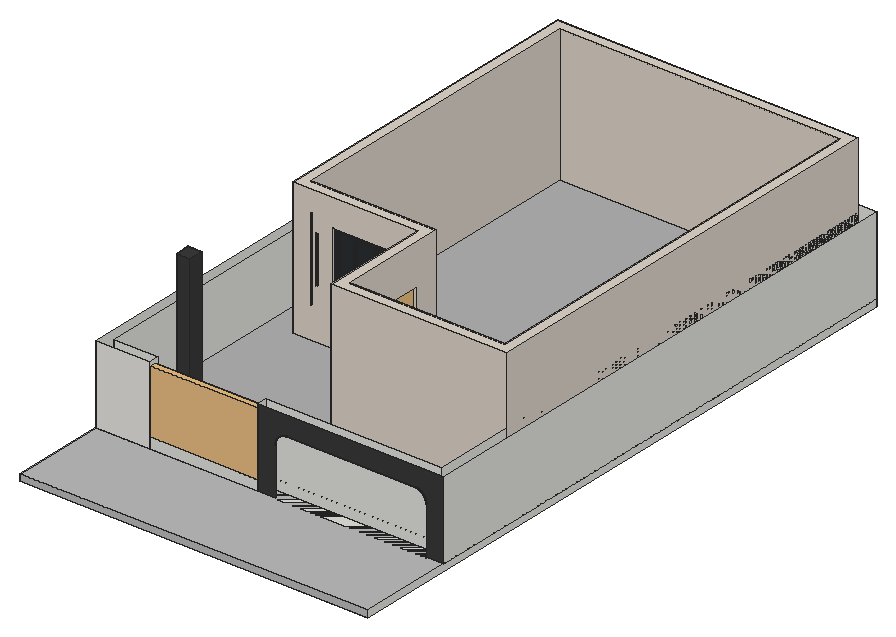
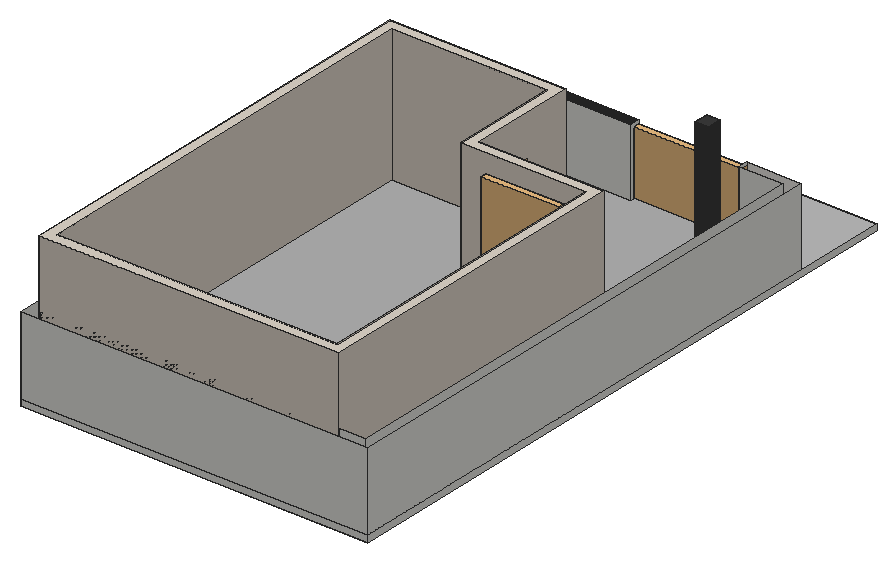
# SketchUp Ruby script. Lengths in inches.
U = 1.inch
M = Sketchup.active_model
def pt(a) = Geom::Point3d.new(a.map { |v| v * U })
def face(e, loops, mat)
  f = e.add_face(loops[0].map { |a| pt(a) })
  loops[1..].each { |l| e.add_face(l.map { |a| pt(a) }).erase! }
  f.material = f.back_material = mat if mat
  f
end
# faces: each face lists its corners as indices into pts; further lists are holes
def faces(e, pts, list, mat = nil) = list.each { |f| face(e, (f[0].is_a?(Array) ? f : [f]).map { |l| l.map { |i| pts[i] } }, mat) }
# xy, xz, yz: faces in a plane at the given z, y or x. An outline is a flat list of corners, or four numbers for a rectangle; further outlines are holes
def ring(l) = l.size == 4 ? [[l[0], l[1]], [l[2], l[1]], [l[2], l[3]], [l[0], l[3]]] : l.each_slice(2).to_a
def flat(e, list, mat, &to3) = list.each { |f| face(e, (f[0].is_a?(Array) ? f : [f]).map { |l| ring(l).map { |u, v| to3.(u, v) } }, mat) }
def xy(e, z, list, mat = nil) = flat(e, list, mat) { |x, y| [x, y, z] }
def xz(e, y, list, mat = nil) = flat(e, list, mat) { |x, z| [x, y, z] }
def yz(e, x, list, mat = nil) = flat(e, list, mat) { |y, z| [x, y, z] }
def lines(e, pts, list) = list.each { |a, b| e.add_line(pt(pts[a]), pt(pts[b])) }
# prism: a flat outline (further loops are holes) pulled along v
def prism(e, loops, v, mat = nil)
  f = face(e, loops, mat); d = Geom::Vector3d.new(v.map { |x| x * U })
  f.pushpull(f.normal.samedirection?(d) ? d.length : -d.length)
end
def box(e, o, s, mat = nil) = prism(e, [[o, [o[0] + s[0], o[1], o[2]], [o[0] + s[0], o[1] + s[1], o[2]], [o[0], o[1] + s[1], o[2]]]], [0, 0, s[2]], mat)
def at(x, y, z, deg = 0) = Geom::Transformation.translation(pt([x, y, z])) * Geom::Transformation.rotation(ORIGIN, Z_AXIS, deg.degrees)
def axes(o, x, y, z) = Geom::Transformation.new([*x, 0, *y, 0, *z, 0, *pt(o).to_a, 1])
def part(name) = M.definitions.add(name)
# library, detail: a bought-in or finely detailed component or shape, given as its bounding box
def library(name, o, s) = part(name).tap { |d| box(d.entities, o, s) }
def detail(e, o, s) = box(e.add_group.entities, o, s)
def put(e, d, t, mat = nil) = e.add_instance(d, t).tap { |i| i.material = mat if mat }
def group(e, t, mat = nil) = e.add_group.tap { |g| g.transformation = t; g.material = mat if mat }.entities
root = M.entities
M.materials.add("1496 AP 8293 CARBON COPY").color = [58, 58, 58]
M.materials.add("1755 AP K184 Brass Olive-N").color = [221, 212, 201]
M.materials.add("Antracyt").color = [44, 47, 50]
M.materials.add("Wall Light").color = [248, 221, 148]
M.materials.add("[Basic Tile]").color = [188, 188, 188]
M.materials.add("[Carrera Marble]").color = [233, 230, 225]
M.materials.add("[Terrazzo Tile Light]").color = [178, 178, 178]
c1 = library("Double slatted gate",[-0.09,68.76,-0.1],[107.6,5.32,60.06])
c2 = part("หน้าต่าง3บาน")
xy(c2.entities,42.78,[[77.6875,12.74,148.55,16.68]],"Antracyt")
xy(c2.entities,43.96,[[78.87,12.74,147.37,12.74,147.37,14.71,125.72,14.71,125.72,13.13,100.52,13.13,100.52,14.71,78.87,14.71],[100.52,13.13,102.88,14.71],[123.36,13.13,125.72,14.71],[102.49,14.71,123.75,14.71,123.75,16.28,147.37,16.28,147.37,16.68,78.87,16.68,78.87,16.28,102.49,16.28]],"Antracyt")
xy(c2.entities,45.93,[[102.49,13.13,123.75,13.92],[102.49,13.92,123.75,14.71],[80.84,14.71,100.52,15.49],[125.72,14.71,145.4,15.49],[80.84,15.49,100.52,16.28],
  [125.72,15.49,145.4,16.28]],"Antracyt")
xy(c2.entities,83.09,[[102.49,13.13,123.75,13.92],[102.49,13.92,123.75,14.71],[80.84,14.71,100.52,15.49],[125.72,14.71,145.4,15.49],[80.84,15.49,100.52,16.28],
  [125.72,15.49,145.4,16.28]],"Antracyt")
xy(c2.entities,84.91,[[78.87,12.74,78.87,14.71,100.52,14.71,100.52,13.13,125.72,13.13,125.72,14.71,147.37,14.71,147.37,12.74],[100.52,13.13,125.72,14.71],[102.49,14.71,102.49,16.28,78.87,16.28,78.87,16.68,147.37,16.68,147.37,16.28,123.75,16.28,123.75,14.71],[78.87,14.71,102.49,16.28]],"Antracyt")
xy(c2.entities,86.09,[[77.6875,12.74,148.55,16.68]],"Antracyt")
xz(c2.entities,12.74,[[[77.6875,42.78,148.55,86.09],[78.87,43.96,147.37,84.91]]],"Antracyt")
xz(c2.entities,13.13,[[[100.52,43.96,125.72,84.91],[102.49,45.93,123.75,83.09]]],"Antracyt")
xz(c2.entities,13.92,[[102.49,45.93,123.75,83.09]],"Antracyt")
xz(c2.entities,14.71,[[78.87,43.96,100.52,43.96,100.52,45.93,80.84,45.93,80.84,83.09,100.52,83.09,100.52,84.91,78.87,84.91],[100.52,43.96,102.49,84.91],[102.49,43.96,123.75,45.93],[125.72,43.96,147.37,43.96,147.37,84.91,125.72,84.91,125.72,83.09,145.4,83.09,145.4,45.93,125.72,45.93],[102.49,83.09,123.75,84.91]],"Antracyt")
xz(c2.entities,15.49,[[80.84,45.93,100.52,83.09],[125.72,45.93,145.4,83.09],[80.44,82.9375,80.84,83.73]],"Antracyt")
xz(c2.entities,16.28,[[[78.87,43.96,102.49,84.91],[80.84,45.93,100.52,83.09]],[[123.75,43.96,147.37,84.91],[125.72,45.93,145.4,83.09]]],"Antracyt")
xz(c2.entities,16.68,[[[77.6875,42.78,148.55,86.09],[78.87,43.96,147.37,84.91]]],"Antracyt")
yz(c2.entities,77.6875,[[12.74,42.78,16.68,86.09]],"Antracyt")
yz(c2.entities,78.87,[[12.74,43.96,14.71,84.91],[16.28,43.96,16.68,84.91]],"Antracyt")
yz(c2.entities,80.84,[[14.71,45.93,15.49,83.09],[15.49,45.93,16.28,83.09]],"Antracyt")
yz(c2.entities,100.52,[[13.13,43.96,14.71,84.91],[14.71,45.93,15.49,83.09],[15.49,45.93,16.28,83.09]],"Antracyt")
yz(c2.entities,102.49,[[14.71,43.96,16.28,84.91],[13.13,45.93,13.92,83.09],[13.92,45.93,14.71,83.09]],"Antracyt")
yz(c2.entities,123.75,[[14.71,43.96,16.28,84.91],[13.13,45.93,13.92,83.09],[13.92,45.93,14.71,83.09]],"Antracyt")
yz(c2.entities,125.72,[[13.13,43.96,14.71,84.91],[14.71,45.93,15.49,83.09],[15.49,45.93,16.28,83.09]],"Antracyt")
yz(c2.entities,145.4,[[14.71,45.93,15.49,83.09],[15.49,45.93,16.28,83.09]],"Antracyt")
yz(c2.entities,147.37,[[12.74,43.96,14.71,84.91],[16.28,43.96,16.68,84.91]],"Antracyt")
yz(c2.entities,148.55,[[12.74,42.78,16.68,86.09]],"Antracyt")
p = [[80.44,15.49,84.91],[80.44,15.49,83.73]]
lines(c2.entities,p,[[0,1]])
c3 = library("Aluprof_MB-86_Drzwi_panelowe_003_S-0452",[0,0,0],[44.84,5.36,87])
c4 = library("Untitled",[23.5,7.18,0],[66.61,8.2,79.03])
box(root,[47,132,9],[12,13,120],"1496 AP 8293 CARBON COPY")
xy(root,0,[[172.5,82.5,172.5,83.5,172.85,83.5,172.85,83.25,173.15,83.25,173.15,83.5,173.5,83.5,173.5,84,158,84,158,93,314,93,314,555,23,555,23,93,62,93,62,84,14,84,14,564,323,564,323,84,307.5,84,307.5,83.5,307.85,83.5,307.85,83.25,308.15,83.25,308.15,83.5,308.5,83.5,308.5,82.5]])
xy(root,52.49,[[183.45,83.5,183.59,84],[297.41,83.5,297.55,84]])
xy(root,52.5,[[183.73,83.5,183.86,84],[183.86,83.5,184,84],[184,83.5,297,84],[297,83.5,297.14,84],[297.14,83.5,297.27,84]])
xz(root,84,[[158,0,173.5,0,173.5,42.27,173.51,42.41,173.51,42.55,173.52,42.6875,173.53,42.82,173.54,42.96,173.56,43.1,173.57,43.23,173.61,43.51,173.63,43.64,173.65,43.78,173.68,43.91,173.7,44.05,173.73,44.18,173.76,44.32,173.82,44.58,173.86,44.72,173.89,44.85,174.01,45.24,174.06,45.375,174.1,45.5,174.3,46.02,174.35,46.14,174.41,46.27,174.46,46.4,174.58,46.64,174.64,46.77,174.71,46.89,174.77,47.01,175.05,47.49,175.12,47.6,175.19,47.72,175.27,47.83,175.35,47.95,175.75,48.5,175.84,48.61,175.93,48.71,176.02,48.82,176.11,48.92,176.2,49.03,176.38,49.23,176.48,49.33,176.58,49.42,176.67,49.52,176.77,49.62,176.97,49.8,177.08,49.89,177.18,49.98,177.29,50.07,177.39,50.16,177.5,50.25,178.05,50.65,178.17,50.73,178.28,50.81,178.4,50.88,178.51,50.95,178.99,51.23,179.11,51.29,179.23,51.36,179.36,51.42,179.6,51.54,179.73,51.59,179.86,51.65,179.98,51.7,180.5,51.9,180.625,51.94,180.76,51.99,181.15,52.11,181.28,52.14,181.42,52.18,181.68,52.24,181.82,52.27,181.95,52.3,182.09,52.32,182.22,52.35,182.36,52.37,182.49,52.39,182.77,52.43,182.9,52.44,183.04,52.46,183.18,52.47,183.3125,52.48,183.45,52.49,183.59,52.49,183.73,52.5,297.27,52.5,297.41,52.49,297.55,52.49,297.6875,52.48,297.82,52.47,297.96,52.46,298.1,52.44,298.23,52.43,298.51,52.39,298.64,52.37,298.78,52.35,298.91,52.32,299.05,52.3,299.18,52.27,299.32,52.24,299.58,52.18,299.72,52.14,299.85,52.11,300.24,51.99,300.375,51.94,300.5,51.9,301.02,51.7,301.14,51.65,301.27,51.59,301.4,51.54,301.64,51.42,301.77,51.36,301.89,51.29,302.01,51.23,302.49,50.95,302.6,50.88,302.72,50.81,302.83,50.73,302.95,50.65,303.5,50.25,303.61,50.16,303.71,50.07,303.82,49.98,303.92,49.89,304.03,49.8,304.23,49.62,304.33,49.52,304.42,49.42,304.52,49.33,304.62,49.23,304.8,49.03,304.89,48.92,304.98,48.82,305.07,48.71,305.16,48.61,305.25,48.5,305.65,47.95,305.73,47.83,305.81,47.72,305.88,47.6,305.95,47.49,306.23,47.01,306.29,46.89,306.36,46.77,306.42,46.64,306.54,46.4,306.59,46.27,306.65,46.14,306.7,46.02,306.9,45.5,306.94,45.375,306.99,45.24,307.11,44.85,307.14,44.72,307.18,44.58,307.24,44.32,307.27,44.18,307.3,44.05,307.32,43.91,307.35,43.78,307.37,43.64,307.39,43.51,307.43,43.23,307.44,43.1,307.46,42.96,307.47,42.82,307.48,42.6875,307.49,42.55,307.49,42.41,307.5,42.27,307.5,0,323,0,323,69,158,69]],"1496 AP 8293 CARBON COPY")
xz(root,84,[[14,0,62,69]],"[Carrera Marble]")
xz(root,93,[[23,0,62,69],[158,0,314,69]])
xz(root,555,[[23,0,314,69]])
xz(root,564,[[14,0,323,69]])
yz(root,14,[[84,0,564,69]])
yz(root,23,[[93,0,555,69]])
yz(root,62,[[84,0,93,69]])
yz(root,158,[[84,0,93,69]])
yz(root,307.49,[[83.5,42.41,84,42.55]])
yz(root,314,[[93,0,555,69]])
yz(root,323,[[84,0,564,69]])
p = [[173.52,84,42.6875],[173.51,84,42.55],[173.51,83.5,42.55],[173.52,83.5,42.6875],[307.49,84,42.55],[307.48,84,42.6875],
  [307.48,83.5,42.6875],[307.49,83.5,42.55],[173.53,84,42.82],[173.53,83.5,42.82],[307.47,84,42.82],[307.47,83.5,42.82],
  [173.54,84,42.96],[173.54,83.5,42.96],[307.46,84,42.96],[307.46,83.5,42.96],[173.56,84,43.1],[173.56,83.5,43.1],
  [307.44,84,43.1],[307.44,83.5,43.1],[173.57,84,43.23],[173.57,83.5,43.23],[307.43,84,43.23],[307.43,83.5,43.23],
  [173.59,84,43.37],[173.59,83.5,43.37],[307.41,84,43.37],[307.41,83.5,43.37],[173.61,84,43.51],[173.61,83.5,43.51],
  [307.39,84,43.51],[307.39,83.5,43.51],[173.63,84,43.64],[173.63,83.5,43.64],[307.37,84,43.64],[307.37,83.5,43.64],
  [173.65,84,43.78],[173.65,83.5,43.78],[307.35,84,43.78],[307.35,83.5,43.78],[173.68,84,43.91],[173.68,83.5,43.91],
  [307.32,84,43.91],[307.32,83.5,43.91],[173.7,84,44.05],[173.7,83.5,44.05],[307.3,84,44.05],[307.3,83.5,44.05],
  [173.73,84,44.18],[173.73,83.5,44.18],[307.27,84,44.18],[307.27,83.5,44.18],[173.76,84,44.32],[173.76,83.5,44.32],
  [307.24,84,44.32],[307.24,83.5,44.32],[173.79,84,44.45],[173.79,83.5,44.45],[307.21,84,44.45],[307.21,83.5,44.45],
  [173.82,84,44.58],[173.82,83.5,44.58],[307.18,84,44.58],[307.18,83.5,44.58],[173.86,84,44.72],[173.86,83.5,44.72],
  [307.14,84,44.72],[307.14,83.5,44.72],[173.89,84,44.85],[173.89,83.5,44.85],[307.11,84,44.85],[307.11,83.5,44.85],
  [173.93,84,44.98],[173.93,83.5,44.98],[307.07,84,44.98],[307.07,83.5,44.98],[173.97,84,45.11],[173.97,83.5,45.11],
  [307.03,84,45.11],[307.03,83.5,45.11],[174.01,84,45.24],[174.01,83.5,45.24],[306.99,84,45.24],[306.99,83.5,45.24],
  [174.06,84,45.375],[174.06,83.5,45.375],[306.94,84,45.375],[306.94,83.5,45.375],[174.1,84,45.5],[174.1,83.5,45.5],
  [306.9,84,45.5],[306.9,83.5,45.5],[174.15,84,45.63],[174.15,83.5,45.63],[306.85,84,45.63],[306.85,83.5,45.63],
  [174.2,84,45.76],[174.2,83.5,45.76],[306.8,84,45.76],[306.8,83.5,45.76],[174.25,84,45.89],[174.25,83.5,45.89],
  [306.75,84,45.89],[306.75,83.5,45.89],[174.3,84,46.02],[174.3,83.5,46.02],[306.7,84,46.02],[306.7,83.5,46.02],
  [174.35,84,46.14],[174.35,83.5,46.14],[306.65,84,46.14],[306.65,83.5,46.14],[174.41,84,46.27],[174.41,83.5,46.27],
  [306.59,84,46.27],[306.59,83.5,46.27],[174.46,84,46.4],[174.46,83.5,46.4],[306.54,84,46.4],[306.54,83.5,46.4],
  [174.52,84,46.52],[174.52,83.5,46.52],[306.48,84,46.52],[306.48,83.5,46.52],[174.58,84,46.64],[174.58,83.5,46.64],
  [306.42,84,46.64],[306.42,83.5,46.64],[174.64,84,46.77],[174.64,83.5,46.77],[306.36,84,46.77],[306.36,83.5,46.77],
  [174.71,84,46.89],[174.71,83.5,46.89],[306.29,84,46.89],[306.29,83.5,46.89],[174.77,84,47.01],[174.77,83.5,47.01],
  [306.23,84,47.01],[306.23,83.5,47.01],[174.84,84,47.13],[174.84,83.5,47.13],[306.16,84,47.13],[306.16,83.5,47.13],
  [174.91,84,47.25],[174.91,83.5,47.25],[306.09,84,47.25],[306.09,83.5,47.25],[306.02,84,47.37],[306.02,83.5,47.37],
  [174.98,84,47.37],[174.98,83.5,47.37],[175.05,84,47.49],[175.05,83.5,47.49],[305.95,84,47.49],[305.95,83.5,47.49],
  [175.12,84,47.6],[175.12,83.5,47.6],[305.88,84,47.6],[305.88,83.5,47.6],[175.19,84,47.72],[175.19,83.5,47.72],
  [305.81,84,47.72],[305.81,83.5,47.72],[175.27,84,47.83],[175.27,83.5,47.83],[305.73,84,47.83],[305.73,83.5,47.83],
  [175.35,84,47.95],[175.35,83.5,47.95],[305.65,84,47.95],[305.65,83.5,47.95],[175.43,84,48.06],[175.43,83.5,48.06],
  [305.57,84,48.06],[305.57,83.5,48.06],[175.51,84,48.17],[175.51,83.5,48.17],[305.49,84,48.17],[305.49,83.5,48.17],
  [175.59,84,48.28],[175.59,83.5,48.28],[305.41,84,48.28],[305.41,83.5,48.28],[175.67,84,48.39],[175.67,83.5,48.39],
  [305.33,84,48.39],[305.33,83.5,48.39],[175.75,84,48.5],[175.75,83.5,48.5],[305.25,84,48.5],[305.25,83.5,48.5],
  [175.84,84,48.61],[175.84,83.5,48.61],[305.16,84,48.61],[305.16,83.5,48.61],[175.93,84,48.71],[175.93,83.5,48.71],
  [305.07,84,48.71],[305.07,83.5,48.71],[176.02,84,48.82],[176.02,83.5,48.82],[304.98,84,48.82],[304.98,83.5,48.82],
  [176.11,84,48.92],[176.11,83.5,48.92],[304.89,84,48.92],[304.89,83.5,48.92],[176.2,84,49.03],[176.2,83.5,49.03],
  [304.8,84,49.03],[304.8,83.5,49.03],[176.29,84,49.13],[176.29,83.5,49.13],[304.71,84,49.13],[304.71,83.5,49.13],
  [176.38,84,49.23],[176.38,83.5,49.23],[304.62,84,49.23],[304.62,83.5,49.23],[176.48,84,49.33],[176.48,83.5,49.33],
  [304.52,84,49.33],[304.52,83.5,49.33],[176.58,84,49.42],[176.58,83.5,49.42],[304.42,84,49.42],[304.42,83.5,49.42],
  [176.67,84,49.52],[176.67,83.5,49.52],[304.33,84,49.52],[304.33,83.5,49.52],[176.77,84,49.62],[176.77,83.5,49.62],
  [304.23,84,49.62],[304.23,83.5,49.62],[176.87,84,49.71],[176.87,83.5,49.71],[304.13,84,49.71],[304.13,83.5,49.71],
  [176.97,84,49.8],[176.97,83.5,49.8],[304.03,84,49.8],[304.03,83.5,49.8],[177.08,84,49.89],[177.08,83.5,49.89],
  [303.92,84,49.89],[303.92,83.5,49.89],[177.18,84,49.98],[177.18,83.5,49.98],[303.82,84,49.98],[303.82,83.5,49.98],
  [177.29,84,50.07],[177.29,83.5,50.07],[303.71,84,50.07],[303.71,83.5,50.07],[177.39,84,50.16],[177.39,83.5,50.16],
  [303.61,84,50.16],[303.61,83.5,50.16],[177.5,84,50.25],[177.5,83.5,50.25],[177.61,84,50.33],[177.61,83.5,50.33],
  [303.5,84,50.25],[303.39,84,50.33],[303.39,83.5,50.33],[303.5,83.5,50.25],[177.72,84,50.41],[177.72,83.5,50.41],
  [303.28,84,50.41],[303.28,83.5,50.41],[177.83,84,50.49],[177.83,83.5,50.49],[303.17,84,50.49],[303.17,83.5,50.49],
  [177.94,84,50.57],[177.94,83.5,50.57],[303.06,84,50.57],[303.06,83.5,50.57],[178.05,84,50.65],[178.05,83.5,50.65],
  [302.95,84,50.65],[302.95,83.5,50.65],[178.17,84,50.73],[178.17,83.5,50.73],[178.28,84,50.81],[178.28,83.5,50.81],
  [302.83,84,50.73],[302.72,84,50.81],[302.72,83.5,50.81],[302.83,83.5,50.73],[178.4,84,50.88],[178.4,83.5,50.88],
  [302.6,84,50.88],[302.6,83.5,50.88],[178.51,84,50.95],[178.51,83.5,50.95],[302.49,84,50.95],[302.49,83.5,50.95],
  [178.63,84,51.02],[178.63,83.5,51.02],[178.75,84,51.09],[178.75,83.5,51.09],[302.37,84,51.02],[302.25,84,51.09],
  [302.25,83.5,51.09],[302.37,83.5,51.02],[178.87,84,51.16],[178.87,83.5,51.16],[302.13,84,51.16],[302.13,83.5,51.16],
  [178.99,84,51.23],[178.99,83.5,51.23],[179.11,84,51.29],[179.11,83.5,51.29],[302.01,84,51.23],[301.89,84,51.29],
  [301.89,83.5,51.29],[302.01,83.5,51.23],[179.23,84,51.36],[179.23,83.5,51.36],[301.77,84,51.36],[301.77,83.5,51.36],
  [179.36,84,51.42],[179.36,83.5,51.42],[179.48,84,51.48],[179.48,83.5,51.48],[301.64,84,51.42],[301.52,84,51.48],
  [301.52,83.5,51.48],[301.64,83.5,51.42],[179.6,84,51.54],[179.6,83.5,51.54],[179.73,84,51.59],[179.73,83.5,51.59],
  [301.4,84,51.54],[301.27,84,51.59],[301.27,83.5,51.59],[301.4,83.5,51.54],[179.86,84,51.65],[179.86,83.5,51.65],
  [179.98,84,51.7],[179.98,83.5,51.7],[301.14,84,51.65],[301.02,84,51.7],[301.02,83.5,51.7],[301.14,83.5,51.65],
  [180.11,84,51.75],[180.11,83.5,51.75],[300.89,84,51.75],[300.89,83.5,51.75],[180.24,84,51.8],[180.24,83.5,51.8],
  [180.37,84,51.85],[180.37,83.5,51.85],[300.76,84,51.8],[300.63,84,51.85],[300.63,83.5,51.85],[300.76,83.5,51.8],
  [180.5,84,51.9],[180.5,83.5,51.9],[180.625,84,51.94],[180.625,83.5,51.94],[180.76,84,51.99],[180.76,83.5,51.99],
  [300.375,84,51.94],[300.24,84,51.99],[300.24,83.5,51.99],[300.375,83.5,51.94],[300.5,84,51.9],[300.5,83.5,51.9],
  [180.89,84,52.03],[180.89,83.5,52.03],[181.02,84,52.07],[181.02,83.5,52.07],[300.11,84,52.03],[299.98,84,52.07],
  [299.98,83.5,52.07],[300.11,83.5,52.03],[181.15,84,52.11],[181.15,83.5,52.11],[181.28,84,52.14],[181.28,83.5,52.14],
  [181.42,84,52.18],[181.42,83.5,52.18],[299.72,84,52.14],[299.58,84,52.18],[299.58,83.5,52.18],[299.72,83.5,52.14],
  [299.85,84,52.11],[299.85,83.5,52.11],[181.55,84,52.21],[181.55,83.5,52.21],[181.68,84,52.24],[181.68,83.5,52.24],
  [181.82,84,52.27],[181.82,83.5,52.27],[299.32,84,52.24],[299.18,84,52.27],[299.18,83.5,52.27],[299.32,83.5,52.24],
  [299.45,84,52.21],[299.45,83.5,52.21],[181.95,84,52.3],[181.95,83.5,52.3],[182.09,84,52.32],[182.09,83.5,52.32],
  [182.22,84,52.35],[182.22,83.5,52.35],[182.36,84,52.37],[182.36,83.5,52.37],[298.78,84,52.35],[298.64,84,52.37],
  [298.64,83.5,52.37],[298.78,83.5,52.35],[298.91,84,52.32],[298.91,83.5,52.32],[299.05,84,52.3],[299.05,83.5,52.3],
  [182.49,84,52.39],[182.49,83.5,52.39],[182.63,84,52.41],[182.63,83.5,52.41],[182.77,84,52.43],[182.77,83.5,52.43],
  [182.9,84,52.44],[182.9,83.5,52.44],[183.04,84,52.46],[183.04,83.5,52.46],[298.1,84,52.44],[297.96,84,52.46],
  [297.96,83.5,52.46],[298.1,83.5,52.44],[298.23,84,52.43],[298.23,83.5,52.43],[298.37,84,52.41],[298.37,83.5,52.41],
  [298.51,84,52.39],[298.51,83.5,52.39],[183.18,84,52.47],[183.18,83.5,52.47],[183.3125,84,52.48],[183.3125,83.5,52.48],
  [183.45,84,52.49],[183.45,83.5,52.49],[183.73,84,52.5],[183.59,84,52.49],[183.59,83.5,52.49],[183.73,83.5,52.5],
  [297.41,84,52.49],[297.27,84,52.5],[297.27,83.5,52.5],[297.41,83.5,52.49],[297.6875,84,52.48],[297.55,84,52.49],
  [297.55,83.5,52.49],[297.6875,83.5,52.48],[297.82,84,52.47],[297.82,83.5,52.47]]
faces(root,p,[[0,1,2,3],[4,5,6,7],[8,0,3,9],[5,10,11,6],[12,8,9,13],[10,14,15,11],[16,12,13,17],[14,18,19,15],
  [20,16,17,21],[18,22,23,19],[24,20,21,25],[22,26,27,23],[28,24,25,29],[26,30,31,27],[32,28,29,33],[30,34,35,31],
  [36,32,33,37],[34,38,39,35],[40,36,37,41],[38,42,43,39],[44,40,41,45],[42,46,47,43],[48,44,45,49],[46,50,51,47],
  [52,48,49,53],[50,54,55,51],[56,52,53,57],[54,58,59,55],[60,56,57,61],[58,62,63,59],[64,60,61,65],[62,66,67,63],
  [68,64,65,69],[66,70,71,67],[72,68,69,73],[70,74,75,71],[76,72,73,77],[74,78,79,75],[80,76,77,81],[78,82,83,79],
  [84,80,81,85],[82,86,87,83],[88,84,85,89],[86,90,91,87],[92,88,89,93],[90,94,95,91],[96,92,93,97],[94,98,99,95],
  [100,96,97,101],[98,102,103,99],[104,100,101,105],[102,106,107,103],[108,104,105,109],[106,110,111,107],[112,108,109,113],[110,114,115,111],
  [116,112,113,117],[114,118,119,115],[120,116,117,121],[118,122,123,119],[124,120,121,125],[122,126,127,123],[128,124,125,129],[126,130,131,127],
  [132,128,129,133],[130,134,135,131],[136,132,133,137],[134,138,139,135],[140,136,137,141],[138,142,143,139],[144,140,141,145],[142,146,147,143],
  [146,148,149,147],[150,144,145,151],[152,150,151,153],[148,154,155,149],[156,152,153,157],[154,158,159,155],[160,156,157,161],[158,162,163,159],
  [164,160,161,165],[162,166,167,163],[168,164,165,169],[166,170,171,167],[172,168,169,173],[170,174,175,171],[176,172,173,177],[174,178,179,175],
  [180,176,177,181],[178,182,183,179],[184,180,181,185],[182,186,187,183],[188,184,185,189],[186,190,191,187],[192,188,189,193],[190,194,195,191],
  [196,192,193,197],[194,198,199,195],[200,196,197,201],[198,202,203,199],[204,200,201,205],[202,206,207,203],[208,204,205,209],[206,210,211,207],
  [212,208,209,213],[210,214,215,211],[216,212,213,217],[214,218,219,215],[220,216,217,221],[218,222,223,219],[224,220,221,225],[222,226,227,223],
  [228,224,225,229],[226,230,231,227],[232,228,229,233],[230,234,235,231],[236,232,233,237],[234,238,239,235],[240,236,237,241],[238,242,243,239],
  [244,240,241,245],[242,246,247,243],[248,244,245,249],[246,250,251,247],[252,248,249,253],[250,254,255,251],[256,252,253,257],[254,258,259,255],
  [260,256,257,261],[262,260,261,263],[264,265,266,267],[258,264,267,259],[268,262,263,269],[265,270,271,266],[272,268,269,273],[270,274,275,271],
  [276,272,273,277],[274,278,279,275],[280,276,277,281],[278,282,283,279],[284,280,281,285],[286,284,285,287],[288,289,290,291],[282,288,291,283],
  [292,286,287,293],[289,294,295,290],[296,292,293,297],[294,298,299,295],[300,296,297,301],[302,300,301,303],[304,305,306,307],[298,304,307,299],
  [308,302,303,309],[305,310,311,306],[312,308,309,313],[314,312,313,315],[316,317,318,319],[310,316,319,311],[320,314,315,321],[317,322,323,318],
  [324,320,321,325],[326,324,325,327],[328,329,330,331],[322,328,331,323],[332,326,327,333],[334,332,333,335],[336,337,338,339],[329,336,339,330],
  [340,334,335,341],[342,340,341,343],[344,345,346,347],[337,344,347,338],[348,342,343,349],[345,350,351,346],[352,348,349,353],[354,352,353,355],
  [356,357,358,359],[350,356,359,351],[360,354,355,361],[362,360,361,363],[364,362,363,365],[366,367,368,369],[370,366,369,371],[357,370,371,358],
  [372,364,365,373],[374,372,373,375],[376,377,378,379],[367,376,379,368],[380,374,375,381],[382,380,381,383],[384,382,383,385],[386,387,388,389],
  [390,386,389,391],[377,390,391,378],[392,384,385,393],[394,392,393,395],[396,394,395,397],[398,399,400,401],[402,398,401,403],[387,402,403,388],
  [404,396,397,405],[406,404,405,407],[408,406,407,409],[410,408,409,411],[412,413,414,415],[416,412,415,417],[418,416,417,419],[399,418,419,400],
  [420,410,411,421],[422,420,421,423],[424,422,423,425],[426,424,425,427],[428,426,427,429],[430,431,432,433],[434,430,433,435],[436,434,435,437],
  [438,436,437,439],[413,438,439,414],[440,428,429,441],[442,440,441,443],[444,442,443,445],[446,447,448,449],[450,451,452,453],[454,455,456,457],
  [458,454,457,459],[431,458,459,432]])
put(root,c1,axes([62.08,158.08,9.1],[0.89216,0,0],[0,-1,0],[0,0,0.95]))
g1 = group(root,at(14,0,-6))
xy(g1,0,[[0,0,309,564]])
xy(g1,6,[[0,0,309,564]],"[Basic Tile]")
xz(g1,0,[[0,0,309,6]],"[Basic Tile]")
xz(g1,564,[[0,0,309,6]])
yz(g1,0,[[0,0,564,6]])
yz(g1,309,[[0,0,564,6]])
g2 = group(root,at(23,93,0))
xy(g2,0,[[39,-9,39,0,0,0,0,462,291,462,291,0,135,0,135,-9]])
xy(g2,9,[[39,-9,135,-9,135,0,291,0,291,462,0,462,0,0,39,0]],"[Terrazzo Tile Light]")
xz(g2,-9,[[39,0,135,9]])
xz(g2,0,[[0,0,39,9],[135,0,291,9]])
xz(g2,462,[[0,0,291,9]])
yz(g2,0,[[0,0,462,9]])
yz(g2,39,[[-9,0,0,9]])
yz(g2,135,[[-9,0,0,9]])
yz(g2,291,[[0,0,462,9]])
g3 = group(root,at(23,165,9))
xy(g3,0,[[135,0,135,42,144,42,144,9,282,9,282,381,33,381,33,105,144,105,144,84,135,84,135,96,24,96,24,390,291,390,291,0]],"1755 AP K184 Brass Olive-N")
xy(g3,28,[[40,96,41,96.5]],"1755 AP K184 Brass Olive-N")
xy(g3,42,[[60,96,114,105]],"1755 AP K184 Brass Olive-N")
xy(g3,45,[[45,96,46,96.5]],"1755 AP K184 Brass Olive-N")
xy(g3,84,[[135,42,144,84]],"1755 AP K184 Brass Olive-N")
xy(g3,87,[[45,96,46,96.5]],"1755 AP K184 Brass Olive-N")
xy(g3,96,[[60,96,114,105]],"1755 AP K184 Brass Olive-N")
xy(g3,102,[[40,96,41,96.5]],"1755 AP K184 Brass Olive-N")
xy(g3,120,[[[135,0,291,0,291,390,24,390,24,96,135,96],[144,9,144,105,33,105,33,381,282,381,282,9]]],"1755 AP K184 Brass Olive-N")
xz(g3,0,[[135,0,291,120]],"1755 AP K184 Brass Olive-N")
xz(g3,9,[[144,0,282,120]],"1755 AP K184 Brass Olive-N")
xz(g3,42,[[135,0,144,84]],"1755 AP K184 Brass Olive-N")
xz(g3,84,[[135,0,144,84]],"1755 AP K184 Brass Olive-N")
xz(g3,96,[[[24,0,135,120],[60,42,114,96],[40,28,41,102],[45,45,46,87]]],"1755 AP K184 Brass Olive-N")
xz(g3,96.5,[[40,28,41,102],[45,45,46,87]],"1755 AP K184 Brass Olive-N")
xz(g3,105,[[[33,0,144,120],[60,42,114,96]]],"1755 AP K184 Brass Olive-N")
xz(g3,381,[[33,0,282,120]],"1755 AP K184 Brass Olive-N")
xz(g3,390,[[24,0,291,120]],"1755 AP K184 Brass Olive-N")
yz(g3,24,[[96,0,390,120]],"1755 AP K184 Brass Olive-N")
yz(g3,33,[[105,0,381,120]],"1755 AP K184 Brass Olive-N")
yz(g3,40,[[96,28,96.5,102]],"1755 AP K184 Brass Olive-N")
yz(g3,41,[[96,28,96.5,102]],"1755 AP K184 Brass Olive-N")
yz(g3,45,[[96,45,96.5,87]],"1755 AP K184 Brass Olive-N")
yz(g3,46,[[96,45,96.5,87]],"1755 AP K184 Brass Olive-N")
yz(g3,60,[[96,42,105,96]],"1755 AP K184 Brass Olive-N")
yz(g3,114,[[96,42,105,96]],"1755 AP K184 Brass Olive-N")
yz(g3,135,[[0,0,0,120,96,120,96,0,84,0,84,84,42,84,42,0]],"1755 AP K184 Brass Olive-N")
yz(g3,144,[[9,0,42,0,42,84,84,84,84,0,105,0,105,120,9,120]],"1755 AP K184 Brass Olive-N")
yz(g3,282,[[9,0,381,120]],"1755 AP K184 Brass Olive-N")
yz(g3,291,[[0,0,390,120]],"1755 AP K184 Brass Olive-N")
put(g3,c2,axes([0.8,84.51,-11.34],[0.762,0,0],[0,1,0],[0,0,1.24691]))
put(g3,c3,axes([135,84,0],[0,-0.93661,0],[1,0,0],[0,0,0.96551]))
put(g3,c4,axes([28.15,100.19,27.32],[1.03545,0,0],[0,0.67,0],[0,0,0.96547]))
g4 = group(g3,at(38,96.5,28),"Wall Light")
box(g4,[2,-0.5,0],[1,0.5,74])
box(g4,[7,-0.5,17],[1,0.5,42])
